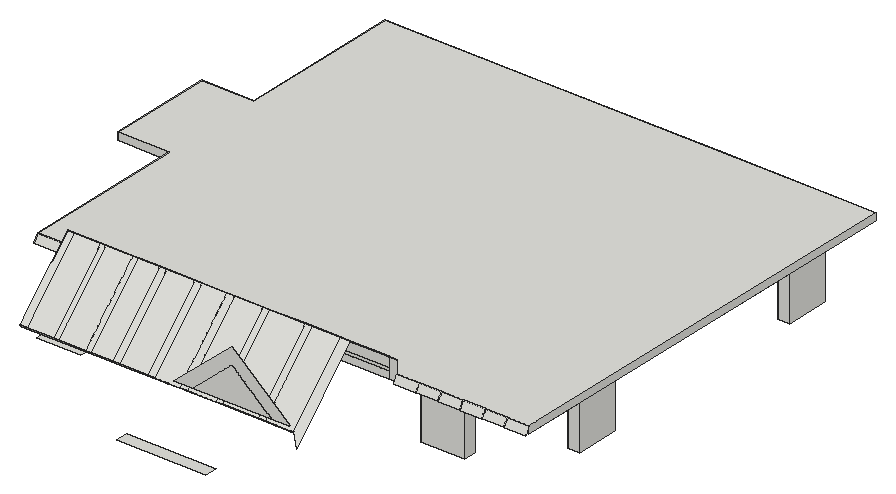
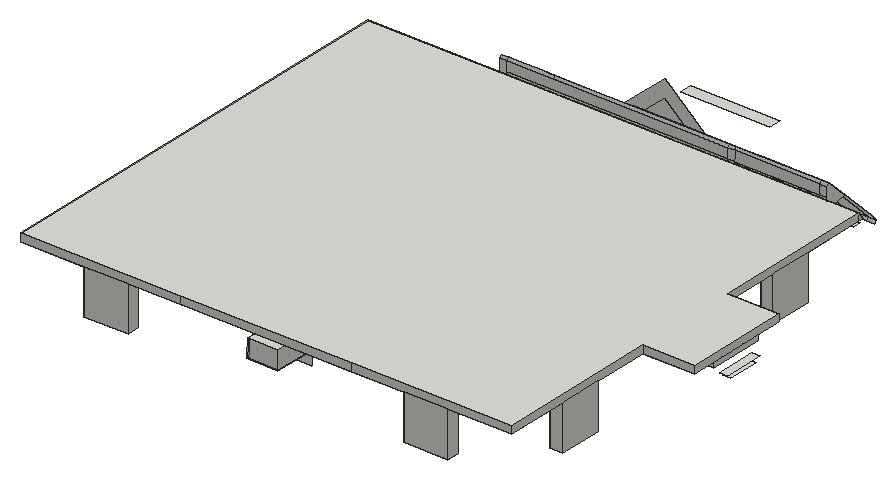
# SketchUp Ruby script. Lengths in inches.
U = 1.inch
M = Sketchup.active_model
def pt(a) = Geom::Point3d.new(a.map { |v| v * U })
def face(e, loops, mat)
  f = e.add_face(loops[0].map { |a| pt(a) })
  loops[1..].each { |l| e.add_face(l.map { |a| pt(a) }).erase! }
  f.material = f.back_material = mat if mat
  f
end
# faces: each face lists its corners as indices into pts; further lists are holes
def faces(e, pts, list, mat = nil) = list.each { |f| face(e, (f[0].is_a?(Array) ? f : [f]).map { |l| l.map { |i| pts[i] } }, mat) }
# xy, xz, yz: faces in a plane at the given z, y or x. An outline is a flat list of corners, or four numbers for a rectangle; further outlines are holes
def ring(l) = l.size == 4 ? [[l[0], l[1]], [l[2], l[1]], [l[2], l[3]], [l[0], l[3]]] : l.each_slice(2).to_a
def flat(e, list, mat, &to3) = list.each { |f| face(e, (f[0].is_a?(Array) ? f : [f]).map { |l| ring(l).map { |u, v| to3.(u, v) } }, mat) }
def xy(e, z, list, mat = nil) = flat(e, list, mat) { |x, y| [x, y, z] }
def xz(e, y, list, mat = nil) = flat(e, list, mat) { |x, z| [x, y, z] }
def yz(e, x, list, mat = nil) = flat(e, list, mat) { |y, z| [x, y, z] }
def lines(e, pts, list) = list.each { |a, b| e.add_line(pt(pts[a]), pt(pts[b])) }
# prism: a flat outline (further loops are holes) pulled along v
def prism(e, loops, v, mat = nil)
  f = face(e, loops, mat); d = Geom::Vector3d.new(v.map { |x| x * U })
  f.pushpull(f.normal.samedirection?(d) ? d.length : -d.length)
end
def box(e, o, s, mat = nil) = prism(e, [[o, [o[0] + s[0], o[1], o[2]], [o[0] + s[0], o[1] + s[1], o[2]], [o[0], o[1] + s[1], o[2]]]], [0, 0, s[2]], mat)
def at(x, y, z, deg = 0) = Geom::Transformation.translation(pt([x, y, z])) * Geom::Transformation.rotation(ORIGIN, Z_AXIS, deg.degrees)
def axes(o, x, y, z) = Geom::Transformation.new([*x, 0, *y, 0, *z, 0, *pt(o).to_a, 1])
def part(name) = M.definitions.add(name)
# library, detail: a bought-in or finely detailed component or shape, given as its bounding box
def library(name, o, s) = part(name).tap { |d| box(d.entities, o, s) }
def detail(e, o, s) = box(e.add_group.entities, o, s)
def put(e, d, t, mat = nil) = e.add_instance(d, t).tap { |i| i.material = mat if mat }
def group(e, t, mat = nil) = e.add_group.tap { |g| g.transformation = t; g.material = mat if mat }.entities
root = M.entities
c1 = part("Agrupar\#13")
detail(c1.entities,[0,0,0],[14.04,13.39,20.05])
c2 = library("Agrupar\#4",[0,0,0],[25,24.8,22.01])
c3 = library("Agrupar\#11",[0,0,0],[3.9375,13.3,10.71])
c4 = library("Agrupar\#17",[0,19.92,0],[16.04,16.04,7.88])
c5 = library("Group\#38",[0,0,0],[13.39,21.1,8.5])
c6 = library("Agrupar\#15",[0,0,0],[14.95,34.1875,20.88])
c7 = library("Group\#40",[0,0,0],[13.39,21.1,8.5])
xy(root,209.125,[[344,206.32,354,242.32]])
xy(root,209.3125,[[84,173.57,94,209.57],[474,173.57,484,209.57]])
xy(root,210,[[245,1.57,317,11.57],[122,73.57,158,79.57]])
xy(root,232.22,[[35.8125,286.57,42,312.5]])
xy(root,235.46,[[35.8125,283.33,42,315.74]])
xy(root,241.6875,[[42,277.1,48,321.97]])
xy(root,246,[[84,118.3125,110,121.57],[84,121.57,136,121.57,136,131.57,94,131.57,94,173.57,84,173.57],[172,121.57,266,131.57],[302,121.57,396,121.57,396,131.57,354,131.57,354,206.32,344,206.32,344,131.57,302,131.57],[432,121.57,484,121.57,484,173.57,474,173.57,474,131.57,432,131.57],
  [84,173.57,94,209.57],[474,173.57,484,209.57],[344,206.32,354,242.32],[84,209.57,94,209.57,94,261.57,48,261.57,48,277.1,42,277.1,42,255.57,84,255.57],[474,209.57,484,209.57,484,387.57,474,387.57,474,261.57,289.625,261.57,289.625,298.57,279.625,298.57,279.625,251.57,474,251.57],
  [344,242.32,354,251.57],[354,242.32,354.45,251.57,354,251.57],[94,251.57,224,261.57],[42,321.97,48,321.97,48,335.57,236.0625,335.57,236.0625,345.57,94,345.57,94,387.57,84,387.57,84,341.57,42,341.57],[272.37,335.57,289.625,335.57,289.625,465.57,279.625,465.57,279.625,345.57,272.37,345.57],
  [84,423.57,94,423.57,94,465.57,136,465.57,136,475.57,84,475.57],[474,423.57,484,423.57,484,475.57,432,475.57,432,465.57,474,465.57],[172,465.57,396,475.57]])
xz(root,73.57,[[229.3,214,281.02,259.3,332.62,214,317.46,214,281.01,246,244.48,214],[244.48,214,281.01,246,317.46,214]])
xz(root,121.57,[[84,246,110,252],[110,246,116,254.0625],[185.11,246,191,254.0625],[371,246,376.6875,262.125],[191,252,371,254.0625],
  [110,254.0625,116,262.125],[116,254.0625,185.11,262.125],[185.11,254.0625,191,262.125],[191,254.0625,371,262.125]])
xz(root,173.57,[[84,209.3125,94,246],[474,209.3125,484,246]])
xz(root,206.32,[[344,209.125,354,246]])
xz(root,209.57,[[84,209.3125,94,246],[474,209.3125,484,246]])
xz(root,242.32,[[344,209.125,354,246]])
xz(root,277.1,[[42,241.6875,48,246]])
xz(root,321.97,[[42,241.6875,48,246]])
xz(root,387.57,[[84,227.66,94,246]])
yz(root,42,[[277.1,241.6875,321.97,246]])
yz(root,48,[[277.1,241.6875,321.97,246]])
yz(root,84,[[173.57,209.3125,209.57,246],[118.3125,246,121.57,252,121.57,246]])
yz(root,94,[[173.57,209.3125,209.57,246]])
yz(root,110,[[118.3125,246,103.58,247.9,119.66,264.02,121.57,262.125,121.57,252],[118.3125,246,121.57,252,121.57,246]])
yz(root,266,[[121.57,209.3125,131.57,246]])
yz(root,344,[[206.32,209.125,242.32,246]])
yz(root,354,[[206.32,209.125,242.32,246]])
yz(root,474,[[173.57,209.3125,209.57,246]])
yz(root,484,[[173.57,209.3125,209.57,246]])
p = [[313.83,422.57,201.16],[313.84,422.59,200.37],[312.66,422.59,200.35],[312.65,422.57,201.13],[312.4,388.47,211.38],[312.65,388.72,200.36],
  [313.83,388.72,200.39],[313.58,388.47,211.41],[313.58,422.32,212.18],[312.4,422.32,212.15],[288.78,422.34,211.61],[289.03,422.59,200.6],
  [332.62,71.66,215.9],[340.12,65.09,209.3125],[340.12,119.66,264.02],[332.62,119.66,264.02],[288.78,353.0625,210.04],[288.76,353.04,210.83],
  [312.38,353.03,211.37],[312.4,353.05,210.58],[290.75,353.0625,210.09],[288.78,353.85,210.0625],[290.75,353.85,210.11],[290.75,359.36,210.23],
  [290.75,360.15,210.25],[290.75,360.54,210.26],[290.75,360.93,210.27],[290.75,361.72,210.28],[288.78,361.72,210.24],[288.78,362.51,210.26],
  [290.75,362.51,210.3],[290.75,364.08,210.34],[290.75,364.87,210.36],[288.78,364.87,210.3125],[288.78,365.66,210.33],[290.75,365.66,210.375],
  [290.75,366.44,210.39],[290.75,366.84,210.4],[290.75,367.23,210.41],[290.75,368.02,210.43],[288.78,368.02,210.38],[288.78,368.81,210.4],
  [290.75,368.8,210.44],[290.75,369.59,210.46],[290.75,369.99,210.47],[290.75,370.38,210.48],[290.75,371.17,210.5],[288.78,371.17,210.45],
  [288.78,371.95,210.47],[290.75,371.95,210.52],[290.75,372.74,210.53],[290.75,373.13,210.54],[290.75,373.53,210.55],[290.75,374.32,210.57],
  [288.78,374.32,210.52],[288.78,375.1,210.54],[290.75,375.1,210.59],[290.75,375.89,210.61],[290.75,376.28,210.61],[290.75,376.68,210.625],
  [290.75,377.46,210.64],[288.78,377.47,210.6],[288.78,378.25,210.61],[290.75,378.25,210.66],[290.75,379.04,210.68],[290.75,379.43,210.6875],
  [290.75,379.83,210.69],[290.75,380.61,210.71],[288.78,380.61,210.67],[288.78,381.4,210.6875],[290.75,381.4,210.73],[290.75,382.1875,210.75],
  [290.75,382.58,210.76],[290.75,382.97,210.77],[290.75,383.76,210.78],[288.78,383.76,210.74],[288.78,384.55,210.76],[290.75,384.55,210.8],
  [290.75,385.34,210.82],[290.75,385.73,210.83],[290.75,386.125,210.84],[290.75,386.91,210.86],[288.78,386.91,210.8125],[288.78,387.7,210.83],
  [312.4,387.6875,211.36],[312.4,371.16,210.99],[312.4,370.37,210.97],[290.75,354.24,210.11],[290.75,354.64,210.125],[290.75,355.42,210.14],
  [288.78,355.42,210.1],[288.78,356.21,210.11],[290.75,356.21,210.16],[290.75,357,210.18],[290.75,357.39,210.1875],[290.75,357.78,210.19],
  [290.75,358.57,210.21],[288.78,358.57,210.17],[288.78,359.36,210.1875],[288.78,354.24,210.07],[288.78,354.64,210.08],[288.78,357.79,210.15],
  [288.78,357,210.13],[288.78,357.39,210.14],[288.77,357.78,210.57],[290.74,357.77,210.62],[288.78,360.15,210.2],[288.78,360.93,210.22],
  [288.78,364.08,210.29],[288.78,366.44,210.35],[288.78,367.23,210.36],[288.78,369.59,210.42],[288.78,370.38,210.4375],[288.78,372.74,210.49],
  [288.78,373.53,210.51],[288.78,375.89,210.5625],[312.38,370.35,211.76],[288.78,376.68,210.58],[288.78,379.04,210.63],[288.78,379.83,210.65],
  [288.78,382.1875,210.7],[288.78,382.98,210.72],[312.06,352.71,225.53],[288.44,352.72,225],[288.76,387.68,211.62],[288.44,387.36,225.78],
  [312.38,387.67,212.15],[312.38,370.74,211.77],[312.38,371.14,211.78],[288.78,385.34,210.78],[288.78,386.125,210.79],[288.78,388.49,210.85],
  [313.56,353.03,211.39],[313.24,352.71,225.56],[313.56,370.35,211.79],[313.24,370.03,225.95],[313.24,369.63,225.94],[313.24,369.24,225.93],
  [312.06,387.35,226.32],[288.76,388.47,211.63],[288.76,422.32,212.4],[288.44,422,226.57],[288.44,388.15,225.8],[312.38,388.46,212.17],
  [312.06,388.13,226.34],[312.38,422.31,212.9375],[312.38,404.99,212.54],[312.38,405.38,212.55],[312.38,405.77,212.5625],[312.4,423.11,212.17],
  [288.78,423.12,211.63],[288.78,457.76,212.42],[312.4,457.75,212.95],[312.4,436.89,212.48],[312.4,436.1,212.46],[312.06,370.03,225.92],
  [312.06,370.42,225.93],[312.06,370.82,225.94],[313.56,371.14,211.8],[313.24,370.82,225.97],[313.56,387.67,212.18],[313.24,387.35,226.34],
  [313.56,388.46,212.2],[313.24,388.13,226.36],[313.56,404.99,212.57],[313.24,404.67,226.74],[313.58,423.11,212.2],[313.56,423.09,212.98],
  [312.38,423.09,212.96],[312.38,436.08,213.25],[313.58,436.1,212.49],[313.56,436.08,213.28],[312.06,421.98,227.1],[288.76,423.1,212.42],
  [288.44,422.78,226.59],[312.06,422.77,227.12],[288.44,457.42,227.37],[288.76,457.74,213.21],[312.38,457.73,213.74],[312.38,436.87,213.27],
  [312.06,404.67,226.71],[312.06,405.45,226.73],[313.58,436.89,212.51],[313.58,457.75,212.98],[313.56,436.87,213.29],[313.56,457.73,213.77],
  [313.56,405.77,212.59],[313.24,405.45,226.76],[313.56,422.3,212.96],[313.24,421.98,227.13],[313.24,422.77,227.15],[313.24,435.76,227.44],
  [312.06,457.41,227.91],[312.06,436.55,227.43],[312.06,435.76,227.42],[313.24,436.55,227.46],[313.24,457.41,227.93],[110,73.57,214],
  [185.07,73.57,214],[185.07,71.66,215.9],[168.39,71.66,215.9],[163.08,71.66,215.9],[141.09,71.66,215.9],[137.55,71.66,215.9],
  [110,71.66,215.9],[185.11,73.57,214],[191,73.57,214],[191,71.66,215.9],[185.11,71.66,215.9],[191.07,73.57,214],
  [191.07,71.66,215.9],[229.3,73.57,214],[229.3,71.66,215.9],[219.58,71.66,215.9],[213.75,71.66,215.9],[244.48,73.57,214],
  [244.48,71.66,215.9],[240.125,71.66,215.9],[317.46,73.57,214],[317.46,71.66,215.9],[309.55,71.66,215.9],[303.72,71.66,215.9],
  [274.83,71.66,215.9],[269,71.66,215.9],[245.96,71.66,215.9],[329.3125,73.57,214],[329.3125,71.66,215.9],[332.62,73.57,214],
  [116,73.64,214.07],[110,73.64,214.07],[110,71.73,215.97],[116,71.73,215.97],[137.55,119.66,264.02],[116,119.66,264.02],
  [116,77.66,221.91],[141.09,119.66,264.02],[163.08,119.66,264.02],[168.39,119.66,264.02],[185.07,119.66,264.02],[185.07,77.66,221.91],
  [191,77.66,221.91],[191,119.66,264.02],[185.11,119.66,264.02],[213.75,119.66,264.02],[219.58,119.66,264.02],[240.125,119.66,264.02],
  [245.96,119.66,264.02],[269,119.66,264.02],[274.83,119.66,264.02],[303.72,119.66,264.02],[309.55,119.66,264.02],[110,119.66,264.02],
  [110,103.58,247.9],[110,77.66,221.91],[312.06,369.64,225.92],[312.06,369.24,225.91],[288.03,351.92,225.76],[288.42,351.92,225.76],
  [312.04,351.91,226.3],[312.04,352.69,226.32],[312.04,458.18,228.71],[298.19,458.18,228.4],[288.03,458.19,228.17],[110,118.3125,246],
  [110,121.57,252],[97,121.57,252],[84,121.57,252],[84,118.3125,246],[376.6875,118.3125,246],[376.875,118.3125,246],
  [376.6875,121.57,252],[394.57,121.57,252],[394.76,118.3125,246],[395.9375,118.3125,246],[395.75,121.57,252],[412.46,121.57,252],
  [412.65,118.3125,246],[413.82,118.3125,246],[413.64,121.57,252],[430.34,121.57,252],[430.53,118.3125,246],[431.71,118.3125,246],
  [431.52,121.57,252],[448.23,121.57,252],[448.42,118.3125,246],[449.59,118.3125,246],[449.41,121.57,252],[466.11,121.57,252],
  [466.3,118.3125,246],[467.48,118.3125,246],[467.29,121.57,252],[484,121.57,252],[484,118.3125,246],[484.1875,118.3125,246],
  [484.08,118.3125,246],[116,121.57,262.125],[110,121.57,262.125],[185.07,121.57,262.125],[191,121.57,262.125],[185.11,121.57,262.125],
  [332.62,121.57,262.125],[371,121.57,262.125],[367.77,119.66,264.02],[371,119.66,264.02],[376.6875,121.57,262.125],[376.6875,119.66,264.02],
  [191.07,79.57,220.02],[191,79.57,220.02],[288.8,359.38,209.11],[312.37,405.37,212.95],[48,321.97,241.6875],[314,321.97,241.6875]]
faces(root,p,[[0,1,2,3],[4,5,6,7],[8,7,6,0],[5,3,0,6],[9,10,11,3],[3,9,8,0],[12,13,14,15],[16,17,18,19,20],
  [16,21,22,20],[23,24,25,26,27,28,29,30,31,32,33,34,35,36,37,38,39,40,41,42,43,44,45,46,47,48,49,50,51,52,53,54,55,56,57,58,59,60,61,62,63,64,65,66,67,68,69,70,71,72,73,74,75,76,77,78,79,80,81,82,83,84,85,86,19,20,22,87,88,89,90,91,92,93,94,95,96,97,98],[21,99,87,22],[99,100,88,87],[100,90,89,88],[101,95,94,93,102,103],[101,97,96,95],[104,101,95,105],
  [98,106,24,23],[107,26,25,24,106],[107,28,27,26],[108,33,32,31],[34,109,36,35],[110,38,37,36,109],[110,40,39,38],[41,111,43,42],
  [112,45,44,43,111],[112,47,46,45],[48,113,50,49],[114,52,51,50,113],[114,54,53,52],[55,115,57,56],[18,19,86,116],[117,59,58,57,115],
  [117,61,60,59],[62,118,64,63],[119,66,65,64,118],[119,68,67,66],[69,120,71,70],[121,73,72,71,120],[121,75,74,73],[122,18,17,123],
  [123,17,124,125],[126,124,17,18,116,127,128],[76,129,78,77],[130,80,79,78,129],[130,82,81,80],[4,131,10,9],[85,128,127,116,86],[122,18,132,133],
  [132,134,135,136,137,133],[18,116,134,132],[9,4,7,8],[138,125,124,126],[139,140,141,142],[143,139,142,144],[145,140,139,143,146,147,148],[149,150,151,152,153,154],
  [116,155,135,134],[116,127,156,155],[157,156,127,128],[157,128,158,159],[158,160,161,159],[128,126,160,158],[126,138,161,160],[144,143,162,163],
  [164,165,163,162],[143,146,164,162],[166,167,168,149],[169,168,149,154],[154,149,166,170],[170,171,167,166],[172,141,140,145],[168,173,174,175],
  [176,174,173,177],[178,177,173,168,169,179],[146,180,165,164],[181,180,146,147,148],[169,154,153,179],[171,170,154,169],[152,178,179,153],[152,153,182,183],
  [182,184,179,153],[183,185,184,182],[181,148,186,187],[187,186,188,189],[148,145,188,186],[145,172,189,188],[175,168,167,190],[190,167,171,191],
  [168,169,171,167],[185,183,152,178],[177,178,192,176],[169,179,193,194],[169,194,191,171],[193,179,184,195],[184,185,196,195],[179,178,185,184],
  [178,192,196,185],[197,198,199,200,201,202,203,204],[205,206,207,208],[198,205,208,199],[206,209,210,207],[209,211,212,213,214,210],[211,215,216,217,212],[215,218,219,220,221,222,223,224,216],
  [218,225,226,219],[225,227,12,226],[228,229,230,231],[204,203,232,233,234,231,230],[203,202,235,232],[202,201,236,235],[201,200,237,236],[238,237,200,199,239],
  [207,240,241,242,238,239,199,208],[210,214,243,241,240,207],[214,213,244,243],[212,217,245,244,213],[216,224,246,245,217],[224,223,247,246],[248,247,223,222],[222,221,249,248],
  [250,249,221,220],[15,250,220,219,226,12],[231,234,233,251,252,253,230],[122,123,125,138,157,156,155,254,255],[255,122,133,137],[256,257,258,259,260,261,262],[144,142,141,172,181,180],[254,255,137,136],
  [155,254,136,135],[138,157,159,161],[180,144,163,165],[175,174,176,192,193,194],[172,181,187,189],[194,175,190,191],[192,193,195,196],[263,264,265,266,267],
  [268,269,270],[271,270,269,272],[272,273,274,271],[275,274,273,276],[276,277,278,275],[279,278,277,280],[280,281,282,279],[283,282,281,284],
  [284,285,286,283],[287,286,285,288],[288,289,290,287],[291,290,289,292],[293,291,292,294],[295,296,251,233],[297,295,233,232,235,236,237,238],[298,299,242,241],
  [299,297,238,242],[300,298,241,243,244,245,246,247,248,249,250,15],[301,300,15,14,302,303],[304,301,303,305]])
lines(root,p,[[306,307],[308,98],[147,309],[310,311]])
put(root,c1,axes([309.16,395.15,200.73],[0.03245,0.58549,0.01142],[-0.34234,0.01822,0.03866],[0.03824,-0.00881,0.34276]))
put(root,c2,axes([309.67,404.27,200.85],[0.02234,0.34032,0.01021],[-0.21294,0.01316,0.02718],[0.03059,-0.00933,0.24418]))
g1 = group(root,at(266,121.57,209.3125))
box(g1,[0,0,0],[36,10,36.6875])
g2 = group(root,at(396,121.57,209.3125))
box(g2,[0,0,0],[36,10,36.6875])
g3 = group(root,at(136,121.57,209.3125))
box(g3,[0,0,0],[36,10,36.6875])
g4 = group(root,at(396,465.57,209.3125))
box(g4,[0,0,0],[36,10,36.6875])
g5 = group(root,at(136,465.57,209.3125))
box(g5,[0,0,0],[36,10,36.6875])
g6 = group(root,at(236.37,335.57,209.3125))
box(g6,[-0.3,0,0],[36.3,10,36.6875])
g7 = group(root,at(94,387.57,209.3125,90))
box(g7,[0,0,0],[36,10,36.6875])
g8 = group(root,at(474,423.57,209.3125,-90))
box(g8,[0,0,0],[36,10,36.6875])
g9 = group(root,at(289.625,299.57,209.3125,90))
box(g9,[0,0,0],[36,10,36.6875])
put(root,c3,axes([306.05,357.69,210.99],[0.04496,1.02439,0.03589],[-1.01052,0.03827,0.17338],[0.17177,-0.04295,1.01061]))
put(root,c4,axes([307.82,393.48,212.48],[-0.72884,0.02761,0.12505],[-0.03243,-0.73884,-0.02589],[0.12389,-0.03098,0.7289]))
put(root,c5,axes([306.41,390.32,217.51],[0.08475,1.93102,0.06766],[-0.55391,0.02098,0.09504],[-0.11478,0.0287,-0.67533]))
put(root,c6,axes([306.28,449.2,213.45],[-0.30771,0.09225,-0.01662],[-0.13019,-0.43394,0.0018],[-0.0219,0.00844,0.45245]))
put(root,c7,axes([296.76,391.78,225.34],[0.72884,-0.02761,-0.12505],[0.04804,1.09462,0.03835],[-0.11888,0.02972,-0.69945]))
g10 = group(root,at(154,261.57,239))
box(g10,[0,0,-1],[36,74,8])
g11 = group(root,at(42,121.57,246))
prism(g11,[[[42,0,0],[42,134,0],[0,134,0],[0,220,0],[42,220,0],[42,354,0],[172,354,0],[312,354,0],[442,354,0],[442,0,0]]],[0,0,6])
